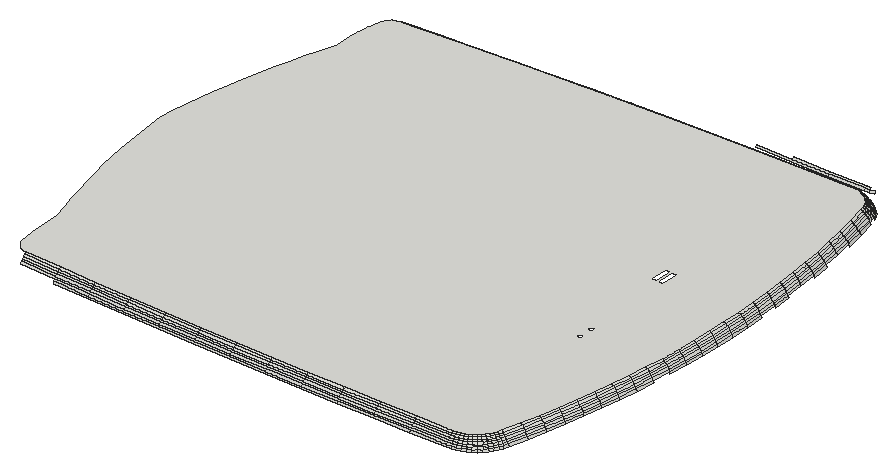
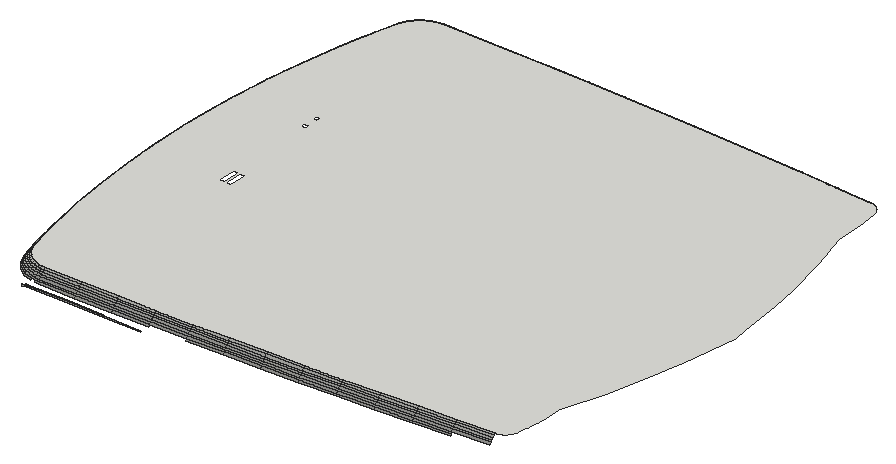
# SketchUp Ruby script. Lengths in inches.
U = 1.inch
M = Sketchup.active_model
def pt(a) = Geom::Point3d.new(a.map { |v| v * U })
def face(e, loops, mat)
  f = e.add_face(loops[0].map { |a| pt(a) })
  loops[1..].each { |l| e.add_face(l.map { |a| pt(a) }).erase! }
  f.material = f.back_material = mat if mat
  f
end
# faces: each face lists its corners as indices into pts; further lists are holes
def faces(e, pts, list, mat = nil) = list.each { |f| face(e, (f[0].is_a?(Array) ? f : [f]).map { |l| l.map { |i| pts[i] } }, mat) }
# xy, xz, yz: faces in a plane at the given z, y or x. An outline is a flat list of corners, or four numbers for a rectangle; further outlines are holes
def ring(l) = l.size == 4 ? [[l[0], l[1]], [l[2], l[1]], [l[2], l[3]], [l[0], l[3]]] : l.each_slice(2).to_a
def flat(e, list, mat, &to3) = list.each { |f| face(e, (f[0].is_a?(Array) ? f : [f]).map { |l| ring(l).map { |u, v| to3.(u, v) } }, mat) }
def xy(e, z, list, mat = nil) = flat(e, list, mat) { |x, y| [x, y, z] }
def xz(e, y, list, mat = nil) = flat(e, list, mat) { |x, z| [x, y, z] }
def yz(e, x, list, mat = nil) = flat(e, list, mat) { |y, z| [x, y, z] }
def lines(e, pts, list) = list.each { |a, b| e.add_line(pt(pts[a]), pt(pts[b])) }
# prism: a flat outline (further loops are holes) pulled along v
def prism(e, loops, v, mat = nil)
  f = face(e, loops, mat); d = Geom::Vector3d.new(v.map { |x| x * U })
  f.pushpull(f.normal.samedirection?(d) ? d.length : -d.length)
end
def box(e, o, s, mat = nil) = prism(e, [[o, [o[0] + s[0], o[1], o[2]], [o[0] + s[0], o[1] + s[1], o[2]], [o[0], o[1] + s[1], o[2]]]], [0, 0, s[2]], mat)
def at(x, y, z, deg = 0) = Geom::Transformation.translation(pt([x, y, z])) * Geom::Transformation.rotation(ORIGIN, Z_AXIS, deg.degrees)
def axes(o, x, y, z) = Geom::Transformation.new([*x, 0, *y, 0, *z, 0, *pt(o).to_a, 1])
def part(name) = M.definitions.add(name)
# library, detail: a bought-in or finely detailed component or shape, given as its bounding box
def library(name, o, s) = part(name).tap { |d| box(d.entities, o, s) }
def detail(e, o, s) = box(e.add_group.entities, o, s)
def put(e, d, t, mat = nil) = e.add_instance(d, t).tap { |i| i.material = mat if mat }
def group(e, t, mat = nil) = e.add_group.tap { |g| g.transformation = t; g.material = mat if mat }.entities
root = M.entities
xy(root,38.7,[[[351.193,51.843,351.37,51.853,351.53,51.881,351.686,51.926,351.836,51.99,351.977,52.07,352.109,52.166,352.228,52.276,352.335,52.399,352.426,52.533,352.502,52.677,352.56,52.829,352.608,53.01,352.823,53.897,353.02,54.788,353.199,55.682,353.359,56.58,353.5,57.481,353.623,58.385,353.726,59.291,353.811,60.199,353.878,61.109,353.925,62.019,353.953,62.931,353.963,63.843,353.953,64.755,353.925,65.666,353.878,66.577,353.811,67.487,353.726,68.395,353.623,69.301,353.5,70.205,353.359,71.106,353.199,72.004,353.02,72.898,352.823,73.788,352.608,74.676,352.56,74.857,352.502,75.009,352.426,75.152,352.335,75.287,352.228,75.41,352.109,75.52,351.977,75.616,351.836,75.696,351.686,75.759,351.53,75.805,351.37,75.833,351.193,75.843,349.441,75.838,347.676,75.824,345.91,75.801,344.144,75.768,342.379,75.726,340.614,75.675,340.613,75.675,338.849,75.615,337.085,75.545,335.321,75.465,333.557,75.377,331.794,75.279,330.048,75.173,329.964,75.162,329.891,75.144,329.82,75.119,329.753,75.086,329.689,75.046,329.63,75,329.576,74.948,329.527,74.891,329.486,74.828,329.451,74.762,329.423,74.692,329.4,74.61,329.364,74.437,329.33,74.254,329.3,74.07,329.275,73.885,329.255,73.7,329.239,73.514,329.228,73.328,329.221,73.141,329.218,72.955,329.221,72.768,329.227,72.582,329.245,72.297,328.999,71.521,328.795,70.834,328.605,70.144,328.428,69.449,328.265,68.752,328.115,68.051,327.978,67.348,327.855,66.642,327.745,65.934,327.649,65.224,327.567,64.513,327.502,63.843,327.567,63.173,327.649,62.461,327.745,61.751,327.855,61.043,327.978,60.338,328.115,59.634,328.265,58.934,328.428,58.236,328.605,57.542,328.795,56.851,328.999,56.165,329.245,55.389,329.227,55.104,329.221,54.917,329.218,54.731,329.221,54.544,329.228,54.358,329.239,54.172,329.255,53.986,329.275,53.801,329.3,53.616,329.33,53.432,329.364,53.249,329.4,53.076,329.423,52.994,329.451,52.924,329.486,52.858,329.527,52.795,329.576,52.738,329.63,52.685,329.689,52.639,329.753,52.6,329.82,52.567,329.891,52.542,329.964,52.524,330.048,52.513,331.794,52.407,333.557,52.309,335.321,52.22,337.085,52.141,338.849,52.071,340.614,52.011,342.379,51.959,344.144,51.917,345.91,51.885,347.676,51.861,349.441,51.847],[350.05,65.612,350.3,66.487],[349.737,65.612,349.987,66.487],[350.378,61.08,350.346,61.085,350.316,61.097,350.29,61.117,350.27,61.143,350.258,61.173,350.253,61.205,350.258,61.238,350.27,61.268,350.29,61.294,350.316,61.314,350.346,61.326,350.378,61.33,350.411,61.326,350.441,61.314,350.467,61.294,350.487,61.268,350.499,61.238,350.503,61.205,350.499,61.173,350.487,61.143,350.467,61.117,350.441,61.097,350.411,61.085],[350.377,60.377,350.344,60.382,350.314,60.394,350.288,60.414,350.268,60.44,350.256,60.47,350.252,60.502,350.256,60.535,350.268,60.565,350.288,60.591,350.314,60.611,350.344,60.623,350.377,60.627,350.409,60.623,350.439,60.611,350.465,60.591,350.485,60.565,350.497,60.535,350.502,60.502,350.497,60.47,350.485,60.44,350.465,60.414,350.439,60.394,350.409,60.382]]])
p = [[349.439,51.479,38.259],[349.439,51.44,38.171],[347.671,51.454,38.171],[347.672,51.493,38.259],[351.204,51.475,38.259],[351.205,51.435,38.171],
  [351.412,51.487,38.259],[351.416,51.447,38.171],[351.613,51.522,38.259],[351.622,51.483,38.171],[344.137,51.549,38.259],[344.136,51.51,38.171],
  [342.368,51.552,38.171],[342.369,51.592,38.259],[345.904,51.517,38.259],[345.903,51.477,38.171],[351.81,51.579,38.259],[351.823,51.542,38.171],
  [351.998,51.659,38.259],[352.016,51.624,38.171],[340.602,51.643,38.259],[340.601,51.603,38.171],[338.834,51.664,38.171],[338.836,51.704,38.259],
  [352.177,51.76,38.259],[352.198,51.727,38.171],[337.069,51.774,38.259],[337.068,51.734,38.171],[335.301,51.813,38.171],[335.303,51.853,38.259],
  [352.342,51.881,38.259],[352.367,51.85,38.171],[333.536,51.902,38.171],[333.538,51.942,38.259],[352.493,52.019,38.259],[352.521,51.992,38.171],
  [331.77,52,38.171],[331.773,52.04,38.259],[352.627,52.174,38.259],[352.658,52.15,38.171],[352.742,52.344,38.259],[352.776,52.323,38.171],
  [352.837,52.525,38.259],[352.874,52.508,38.171],[352.911,52.716,38.259],[352.949,52.704,38.171],[352.964,52.92,38.259],[353.003,52.91,38.171],
  [353.182,53.814,38.259],[353.221,53.805,38.171],[353.38,54.712,38.259],[353.419,54.704,38.171],[353.56,55.614,38.259],[353.6,55.607,38.171],
  [353.722,56.519,38.259],[353.761,56.513,38.171],[353.864,57.428,38.259],[353.904,57.422,38.171],[353.988,58.339,38.259],[354.027,58.334,38.171],
  [354.092,59.253,38.259],[354.132,59.249,38.171],[354.178,60.168,38.259],[354.218,60.165,38.171],[354.292,62.004,38.259],[354.332,62.002,38.171],
  [354.285,61.083,38.171],[354.245,61.086,38.259],[354.321,62.923,38.259],[354.361,62.922,38.171],[354.331,63.843,38.259],[354.37,63.843,38.171],
  [354.321,64.762,38.259],[354.361,64.763,38.171],[354.292,65.682,38.259],[354.332,65.683,38.171],[354.245,66.6,38.259],[354.285,66.603,38.171],
  [354.092,68.433,38.259],[354.132,68.437,38.171],[354.218,67.521,38.171],[354.178,67.517,38.259],[353.722,71.166,38.259],[353.761,71.173,38.171],
  [353.904,70.264,38.171],[353.864,70.258,38.259],[353.182,73.872,38.259],[353.221,73.881,38.171],[353.419,72.982,38.171],[353.38,72.974,38.259],
  [352.964,74.766,38.259],[353.003,74.775,38.171],[352.742,75.342,38.259],[352.776,75.363,38.171],[352.874,75.177,38.171],[352.837,75.161,38.259],
  [352.627,75.511,38.259],[352.658,75.536,38.171],[352.493,75.666,38.259],[352.521,75.694,38.171],[331.773,75.646,38.259],[331.77,75.686,38.171],
  [333.536,75.784,38.171],[333.538,75.744,38.259],[335.301,75.873,38.171],[335.303,75.833,38.259],[352.342,75.805,38.259],[352.367,75.836,38.171],
  [337.068,75.952,38.171],[337.069,75.912,38.259],[352.177,75.926,38.259],[352.198,75.959,38.171],[338.834,76.022,38.171],[338.836,75.982,38.259],
  [351.998,76.026,38.259],[352.016,76.062,38.171],[340.601,76.083,38.171],[340.602,76.043,38.259],[342.368,76.134,38.171],[342.369,76.094,38.259],
  [351.81,76.106,38.259],[351.823,76.144,38.171],[344.136,76.176,38.171],[344.137,76.136,38.259],[351.613,76.164,38.259],[351.622,76.203,38.171],
  [345.904,76.169,38.259],[345.903,76.209,38.171],[347.671,76.232,38.171],[347.672,76.192,38.259],[349.439,76.246,38.171],[349.439,76.206,38.259],
  [351.205,76.251,38.171],[351.204,76.211,38.259],[351.416,76.239,38.171],[351.412,76.199,38.259],[347.672,76.743,38.259],[347.671,76.704,38.171],
  [345.903,76.727,38.171],[345.904,76.767,38.259],[349.439,76.729,38.259],[349.439,76.69,38.171],[351.204,76.725,38.259],[351.205,76.685,38.171],
  [351.412,76.737,38.259],[351.416,76.697,38.171],[351.613,76.772,38.259],[351.622,76.733,38.171],[344.138,51.596,38.344],[342.371,51.638,38.344],
  [345.905,51.563,38.344],[347.672,51.54,38.344],[347.673,51.593,38.424],[345.906,51.616,38.424],[349.44,51.526,38.344],[349.44,51.579,38.424],
  [351.202,51.521,38.344],[351.201,51.574,38.424],[351.406,51.533,38.344],[351.4,51.586,38.424],[351.603,51.567,38.344],[351.591,51.619,38.424],
  [351.794,51.623,38.344],[340.604,51.689,38.344],[338.837,51.75,38.344],[342.372,51.691,38.424],[340.605,51.742,38.424],[344.139,51.649,38.424],
  [351.776,51.673,38.424],[351.978,51.701,38.344],[351.954,51.749,38.424],[337.071,51.82,38.344],[338.839,51.803,38.424],[337.073,51.873,38.424],
  [352.151,51.799,38.344],[352.123,51.844,38.424],[335.305,51.899,38.344],[335.308,51.952,38.424],[352.279,51.958,38.424],[352.3125,51.917,38.344],
  [333.54,51.988,38.344],[331.775,52.086,38.344],[333.543,52.041,38.424],[352.459,52.052,38.344],[352.421,52.089,38.424],[331.778,52.139,38.424],
  [352.59,52.203,38.344],[330.017,52.193,38.344],[330.022,52.246,38.424],[352.548,52.235,38.424],[352.657,52.395,38.424],[352.702,52.367,38.344],
  [352.795,52.544,38.344],[352.747,52.566,38.424],[352.816,52.746,38.424],[352.867,52.73,38.344],[352.868,52.944,38.424],[352.919,52.932,38.344],
  [353.136,53.825,38.344],[353.085,53.837,38.424],[353.335,54.722,38.344],[353.283,54.732,38.424],[353.515,55.623,38.344],[353.463,55.632,38.424],
  [353.676,56.527,38.344],[353.624,56.536,38.424],[353.766,57.442,38.424],[353.818,57.435,38.344],[353.942,58.345,38.344],[353.889,58.351,38.424],
  [354.046,59.258,38.344],[353.994,59.263,38.424],[354.132,60.172,38.344],[354.079,60.177,38.424],[354.198,61.089,38.344],[354.146,61.092,38.424],
  [354.193,62.008,38.424],[354.246,62.006,38.344],[354.275,62.924,38.344],[354.222,62.925,38.424],[354.231,63.843,38.424],[354.284,63.843,38.344],
  [354.222,64.76,38.424],[354.275,64.762,38.344],[354.193,65.678,38.424],[354.246,65.68,38.344],[354.146,66.594,38.424],[354.198,66.597,38.344],
  [354.079,67.509,38.424],[354.132,67.513,38.344],[353.994,68.423,38.424],[354.046,68.428,38.344],[353.889,69.334,38.424],[353.942,69.341,38.344],
  [353.988,69.347,38.259],[353.766,70.244,38.424],[353.818,70.251,38.344],[353.624,71.15,38.424],[353.676,71.159,38.344],[353.463,72.053,38.424],
  [353.515,72.063,38.344],[353.56,72.072,38.259],[353.283,72.953,38.424],[353.335,72.964,38.344],[353.085,73.849,38.424],[353.136,73.861,38.344],
  [352.868,74.741,38.424],[352.919,74.754,38.344],[352.816,74.939,38.424],[352.867,74.956,38.344],[352.911,74.97,38.259],[352.747,75.12,38.424],
  [352.795,75.142,38.344],[352.657,75.291,38.424],[352.702,75.318,38.344],[352.548,75.451,38.424],[352.59,75.483,38.344],[330.022,75.44,38.424],
  [330.017,75.493,38.344],[331.775,75.6,38.344],[331.778,75.547,38.424],[333.54,75.698,38.344],[333.543,75.645,38.424],[352.421,75.597,38.424],
  [352.459,75.634,38.344],[335.305,75.786,38.344],[335.308,75.734,38.424],[352.279,75.728,38.424],[352.3125,75.769,38.344],[337.071,75.866,38.344],
  [337.073,75.813,38.424],[352.123,75.842,38.424],[352.151,75.886,38.344],[338.837,75.936,38.344],[338.839,75.883,38.424],[351.954,75.937,38.424],
  [351.978,75.985,38.344],[340.603,75.996,38.344],[340.605,75.944,38.424],[342.371,76.048,38.344],[342.372,75.995,38.424],[351.776,76.013,38.424],
  [351.794,76.0625,38.344],[344.138,76.09,38.344],[344.139,76.037,38.424],[345.905,76.122,38.344],[345.906,76.07,38.424],[351.591,76.067,38.424],
  [351.603,76.119,38.344],[347.672,76.146,38.344],[347.673,76.093,38.424],[349.44,76.16,38.344],[349.44,76.107,38.424],[351.202,76.164,38.344],
  [351.201,76.112,38.424],[351.406,76.153,38.344],[351.4,76.1,38.424],[349.44,76.776,38.344],[347.672,76.79,38.344],[351.202,76.771,38.344],
  [351.406,76.783,38.344],[344.14,51.708,38.501],[342.374,51.75,38.501],[345.907,51.675,38.501],[347.673,51.652,38.501],[349.44,51.638,38.501],
  [351.199,51.633,38.501],[351.393,51.644,38.501],[351.577,51.676,38.501],[351.756,51.729,38.501],[340.607,51.801,38.501],[338.841,51.862,38.501],
  [351.928,51.802,38.501],[352.091,51.893,38.501],[337.076,51.932,38.501],[352.242,52.003,38.501],[335.311,52.011,38.501],[333.546,52.1,38.501],
  [331.782,52.198,38.501],[352.379,52.13,38.501],[330.028,52.304,38.501],[352.501,52.271,38.501],[352.606,52.425,38.501],[352.693,52.59,38.501],
  [352.76,52.764,38.501],[352.811,52.959,38.501],[353.028,53.85,38.501],[353.226,54.745,38.501],[353.405,55.643,38.501],[353.566,56.545,38.501],
  [353.708,57.451,38.501],[353.831,58.359,38.501],[353.935,59.269,38.501],[354.02,60.182,38.501],[354.087,61.096,38.501],[354.134,62.011,38.501],
  [354.163,62.927,38.501],[354.172,63.843,38.501],[354.163,64.759,38.501],[354.134,65.675,38.501],[354.087,66.59,38.501],[354.02,67.504,38.501],
  [353.935,68.417,38.501],[353.831,69.327,38.501],[353.708,70.235,38.501],[353.566,71.14,38.501],[353.405,72.042,38.501],[353.226,72.941,38.501],
  [353.028,73.836,38.501],[352.811,74.727,38.501],[352.76,74.921,38.501],[352.693,75.095,38.501],[352.606,75.261,38.501],[352.501,75.415,38.501],
  [330.028,75.381,38.501],[331.782,75.488,38.501],[352.379,75.556,38.501],[333.546,75.586,38.501],[335.311,75.675,38.501],[352.242,75.682,38.501],
  [337.076,75.754,38.501],[352.091,75.792,38.501],[338.841,75.824,38.501],[340.607,75.885,38.501],[351.928,75.884,38.501],[342.374,75.936,38.501],
  [344.14,75.978,38.501],[351.756,75.957,38.501],[345.907,76.011,38.501],[347.673,76.034,38.501],[349.44,76.048,38.501],[351.199,76.053,38.501],
  [351.393,76.042,38.501],[351.577,76.01,38.501],[349.441,51.702,38.573],[347.674,51.716,38.573],[351.197,51.698,38.573],[351.386,51.709,38.573],
  [351.5625,51.739,38.573],[342.375,51.814,38.573],[340.609,51.866,38.573],[344.141,51.772,38.573],[345.908,51.74,38.573],[351.735,51.79,38.573],
  [351.9,51.86,38.573],[338.844,51.926,38.573],[352.056,51.948,38.573],[337.079,51.996,38.573],[335.314,52.076,38.573],[352.201,52.053,38.573],
  [333.549,52.164,38.573],[352.332,52.175,38.573],[331.786,52.262,38.573],[352.45,52.31,38.573],[330.034,52.369,38.573],[352.551,52.459,38.573],
  [352.634,52.617,38.573],[352.699,52.784,38.573],[352.748,52.975,38.573],[352.965,53.865,38.573],[353.162,54.758,38.573],[353.341,55.655,38.573],
  [353.502,56.556,38.573],[353.644,57.46,38.573],[353.767,58.367,38.573],[353.871,59.276,38.573],[353.956,60.187,38.573],[354.022,61.1,38.573],
  [354.07,62.013,38.573],[354.098,62.928,38.573],[354.108,63.843,38.573],[354.098,64.758,38.573],[354.07,65.672,38.573],[354.022,66.586,38.573],
  [353.956,67.499,38.573],[353.871,68.41,38.573],[353.767,69.319,38.573],[353.644,70.226,38.573],[353.502,71.13,38.573],[353.341,72.03,38.573],
  [353.162,72.928,38.573],[352.965,73.821,38.573],[352.748,74.711,38.573],[352.699,74.901,38.573],[352.634,75.069,38.573],[352.551,75.227,38.573],
  [352.45,75.375,38.573],[330.034,75.317,38.573],[331.786,75.424,38.573],[333.549,75.522,38.573],[352.332,75.511,38.573],[335.314,75.61,38.573],
  [352.201,75.632,38.573],[337.079,75.689,38.573],[352.056,75.738,38.573],[338.844,75.759,38.573],[351.9,75.826,38.573],[340.608,75.82,38.573],
  [342.375,75.871,38.573],[351.735,75.896,38.573],[344.141,75.913,38.573],[345.908,75.946,38.573],[347.674,75.969,38.573],[351.386,75.977,38.573],
  [351.5625,75.947,38.573],[349.441,75.983,38.573],[351.197,75.988,38.573],[345.909,51.81,38.639],[344.143,51.842,38.639],[347.675,51.786,38.639],
  [349.441,51.772,38.639],[351.196,51.768,38.639],[351.378,51.778,38.639],[351.547,51.807,38.639],[351.711,51.856,38.639],[342.377,51.884,38.639],
  [340.612,51.936,38.639],[344.144,51.917,38.7],[342.379,51.959,38.7],[345.91,51.885,38.7],[347.676,51.861,38.7],[349.441,51.847,38.7],
  [351.193,51.843,38.7],[351.37,51.853,38.7],[351.53,51.881,38.7],[351.686,51.926,38.7],[351.869,51.923,38.639],[338.846,51.996,38.639],
  [337.082,52.066,38.639],[340.614,52.011,38.7],[338.849,52.071,38.7],[351.836,51.99,38.7],[351.977,52.07,38.7],[352.018,52.007,38.639],
  [352.156,52.108,38.639],[335.317,52.146,38.639],[337.085,52.141,38.7],[352.109,52.166,38.7],[333.553,52.234,38.639],[335.321,52.22,38.7],
  [333.557,52.309,38.7],[352.228,52.276,38.7],[352.282,52.224,38.639],[331.79,52.332,38.639],[331.794,52.407,38.7],[352.335,52.399,38.7],
  [352.394,52.353,38.639],[330.041,52.438,38.639],[330.048,52.513,38.7],[352.49,52.495,38.639],[352.426,52.533,38.7],[352.502,52.677,38.7],
  [352.57,52.646,38.639],[352.56,52.829,38.7],[352.632,52.806,38.639],[352.68,52.992,38.639],[352.608,53.01,38.7],[352.823,53.897,38.7],
  [352.896,53.88,38.639],[353.02,54.788,38.7],[353.094,54.772,38.639],[353.199,55.682,38.7],[353.273,55.668,38.639],[353.359,56.58,38.7],
  [353.433,56.568,38.639],[353.574,57.47,38.639],[353.5,57.481,38.7],[353.623,58.385,38.7],[353.697,58.375,38.639],[353.726,59.291,38.7],
  [353.801,59.283,38.639],[353.811,60.199,38.7],[353.886,60.193,38.639],[353.878,61.109,38.7],[353.952,61.104,38.639],[353.925,62.019,38.7],
  [354,62.016,38.639],[353.953,62.931,38.7],[354.028,62.929,38.639],[354.038,63.843,38.639],[353.963,63.843,38.7],[353.953,64.755,38.7],
  [354.028,64.756,38.639],[353.925,65.666,38.7],[354,65.67,38.639],[353.878,66.577,38.7],[353.952,66.582,38.639],[353.811,67.487,38.7],
  [353.886,67.493,38.639],[353.726,68.395,38.7],[353.801,68.403,38.639],[353.623,69.301,38.7],[353.697,69.31,38.639],[353.5,70.205,38.7],
  [353.574,70.216,38.639],[353.359,71.106,38.7],[353.433,71.118,38.639],[353.199,72.004,38.7],[353.273,72.017,38.639],[353.02,72.898,38.7],
  [353.094,72.913,38.639],[352.823,73.788,38.7],[352.896,73.805,38.639],[352.608,74.676,38.7],[352.68,74.694,38.639],[352.56,74.857,38.7],
  [352.632,74.88,38.639],[352.502,75.009,38.7],[352.57,75.04,38.639],[352.426,75.152,38.7],[352.49,75.191,38.639],[330.048,75.173,38.7],
  [330.041,75.247,38.639],[331.79,75.354,38.639],[331.794,75.279,38.7],[352.335,75.287,38.7],[352.394,75.333,38.639],[333.553,75.452,38.639],
  [333.557,75.377,38.7],[352.228,75.41,38.7],[352.282,75.462,38.639],[335.317,75.54,38.639],[335.321,75.465,38.7],[352.109,75.52,38.7],
  [352.156,75.578,38.639],[337.082,75.619,38.639],[337.085,75.545,38.7],[338.846,75.689,38.639],[338.849,75.615,38.7],[351.977,75.616,38.7],
  [352.018,75.679,38.639],[340.61,75.75,38.639],[340.613,75.675,38.7],[351.836,75.696,38.7],[351.869,75.763,38.639],[342.379,75.726,38.7],
  [340.614,75.675,38.7],[340.612,75.75,38.639],[342.377,75.801,38.639],[344.143,75.843,38.639],[344.144,75.768,38.7],[351.686,75.759,38.7],
  [351.711,75.83,38.639],[345.909,75.876,38.639],[345.91,75.801,38.7],[347.675,75.899,38.639],[347.676,75.824,38.7],[349.441,75.913,38.639],
  [349.441,75.838,38.7],[351.196,75.918,38.639],[351.193,75.843,38.7],[351.378,75.908,38.639],[351.37,75.833,38.7],[351.547,75.878,38.639],
  [351.53,75.805,38.7]]
faces(root,p,[[0,1,2,3],[4,5,1,0],[6,7,5,4],[8,9,7,6],[10,11,12,13],[14,15,11,10],[3,2,15,14],[16,17,9,8],
  [18,19,17,16],[20,21,22,23],[13,12,21,20],[24,25,19,18],[26,27,28,29],[23,22,27,26],[30,31,25,24],[29,28,32,33],
  [34,35,31,30],[33,32,36,37],[38,39,35,34],[40,41,39,38],[42,43,41,40],[44,45,43,42],[46,47,45,44],[48,49,47,46],
  [50,51,49,48],[52,53,51,50],[54,55,53,52],[56,57,55,54],[58,59,57,56],[60,61,59,58],[62,63,61,60],[64,65,66,67],
  [68,69,65,64],[70,71,69,68],[72,73,71,70],[74,75,73,72],[76,77,75,74],[78,79,80,81],[82,83,84,85],[86,87,88,89],
  [90,91,87,86],[92,93,94,95],[96,97,93,92],[98,99,97,96],[100,101,102,103],[103,102,104,105],[106,107,99,98],[105,104,108,109],
  [110,111,107,106],[109,108,112,113],[114,115,111,110],[113,112,116,117],[117,116,118,119],[120,121,115,114],[119,118,122,123],[124,125,121,120],
  [126,127,128,129],[129,128,130,131],[131,130,132,133],[133,132,134,135],[136,137,138,139],[140,141,137,136],[142,143,141,140],[144,145,143,142],
  [146,147,145,144],[148,10,13,149],[150,14,10,148],[151,3,14,150],[152,151,150,153],[154,0,3,151],[155,154,151,152],[156,4,0,154],
  [157,156,154,155],[158,6,4,156],[159,158,156,157],[160,8,6,158],[161,160,158,159],[162,16,8,160],[163,20,23,164],[149,13,20,163],
  [165,149,163,166],[167,148,149,165],[153,150,148,167],[168,162,160,161],[169,18,16,162],[170,169,162,168],[164,23,26,171],[172,164,171,173],
  [166,163,164,172],[174,24,18,169],[175,174,169,170],[171,26,29,176],[173,171,176,177],[178,179,174,175],[179,30,24,174],[180,33,37,181],
  [176,29,33,180],[177,176,180,182],[183,34,30,179],[184,183,179,178],[182,180,181,185],[186,38,34,183],[185,181,187,188],[189,186,183,184],
  [190,191,186,189],[191,40,38,186],[192,42,40,191],[193,192,191,190],[194,195,192,193],[195,44,42,192],[196,197,195,194],[197,46,44,195],
  [198,48,46,197],[199,198,197,196],[200,50,48,198],[201,200,198,199],[202,52,50,200],[203,202,200,201],[204,54,52,202],[205,204,202,203],
  [206,207,204,205],[207,56,54,204],[208,58,56,207],[209,208,207,206],[210,60,58,208],[211,210,208,209],[212,62,60,210],[213,212,210,211],
  [214,67,62,212],[215,214,212,213],[216,217,214,215],[217,64,67,214],[218,68,64,217],[219,218,217,216],[220,221,218,219],[221,70,68,218],
  [222,223,221,220],[223,72,70,221],[224,225,223,222],[225,74,72,223],[226,227,225,224],[227,76,74,225],[228,229,227,226],[229,81,76,227],
  [230,231,229,228],[231,78,81,229],[232,233,231,230],[233,234,78,231],[235,236,233,232],[236,85,234,233],[237,238,236,235],[238,82,85,236],
  [239,240,238,237],[240,241,82,238],[242,243,240,239],[243,89,241,240],[244,245,243,242],[245,86,89,243],[246,247,245,244],[247,90,86,245],
  [248,249,247,246],[249,250,90,247],[251,252,249,248],[252,95,250,249],[253,254,252,251],[254,92,95,252],[255,256,254,253],[256,96,92,254],
  [257,258,259,260],[260,259,261,262],[263,264,256,255],[264,98,96,256],[259,100,103,261],[262,261,265,266],[267,268,264,263],[268,106,98,264],
  [261,103,105,265],[266,265,269,270],[271,272,268,267],[265,105,109,269],[270,269,273,274],[275,276,272,271],[272,110,106,268],[269,109,113,273],
  [274,273,277,278],[273,113,117,277],[278,277,279,280],[281,282,276,275],[276,114,110,272],[277,117,119,279],[280,279,283,284],[279,119,123,283],
  [284,283,285,286],[287,288,282,281],[282,120,114,276],[283,123,126,285],[286,285,289,290],[285,126,129,289],[290,289,291,292],[289,129,131,291],
  [292,291,293,294],[294,293,295,296],[296,295,288,287],[295,135,124,288],[288,124,120,282],[291,131,133,293],[293,133,135,295],[297,140,136,298],
  [299,142,140,297],[300,144,142,299],[301,167,165,302],[303,153,167,301],[304,152,153,303],[305,155,152,304],[306,157,155,305],[307,159,157,306],
  [308,161,159,307],[309,168,161,308],[310,166,172,311],[302,165,166,310],[312,170,168,309],[313,175,170,312],[311,172,173,314],[315,178,175,313],
  [314,173,177,316],[317,182,185,318],[316,177,182,317],[319,184,178,315],[318,185,188,320],[321,189,184,319],[322,190,189,321],[323,193,190,322],
  [324,194,193,323],[325,196,194,324],[326,199,196,325],[327,201,199,326],[328,203,201,327],[329,205,203,328],[330,206,205,329],[331,209,206,330],
  [332,211,209,331],[333,213,211,332],[334,215,213,333],[335,216,215,334],[336,219,216,335],[337,220,219,336],[338,222,220,337],[339,224,222,338],
  [340,226,224,339],[341,228,226,340],[342,230,228,341],[343,232,230,342],[344,235,232,343],[345,237,235,344],[346,239,237,345],[347,242,239,346],
  [348,244,242,347],[349,246,244,348],[350,248,246,349],[351,251,248,350],[352,253,251,351],[353,255,253,352],[354,257,260,355],[356,263,255,353],
  [355,260,262,357],[357,262,266,358],[359,267,263,356],[358,266,270,360],[361,271,267,359],[360,270,274,362],[362,274,278,363],[364,275,271,361],
  [363,278,280,365],[365,280,284,366],[367,281,275,364],[366,284,286,368],[368,286,290,369],[369,290,292,370],[370,292,294,371],[371,294,296,372],
  [372,296,287,373],[373,287,281,367],[374,305,304,375],[376,306,305,374],[377,307,306,376],[378,308,307,377],[379,302,310,380],[381,301,302,379],
  [382,303,301,381],[375,304,303,382],[383,309,308,378],[384,312,309,383],[380,310,311,385],[386,313,312,384],[387,314,316,388],[385,311,314,387],
  [389,315,313,386],[388,316,317,390],[391,319,315,389],[390,317,318,392],[393,321,319,391],[392,318,320,394],[395,322,321,393],[396,323,322,395],
  [397,324,323,396],[398,325,324,397],[399,326,325,398],[400,327,326,399],[401,328,327,400],[402,329,328,401],[403,330,329,402],[404,331,330,403],
  [405,332,331,404],[406,333,332,405],[407,334,333,406],[408,335,334,407],[409,336,335,408],[410,337,336,409],[411,338,337,410],[412,339,338,411],
  [413,340,339,412],[414,341,340,413],[415,342,341,414],[416,343,342,415],[417,344,343,416],[418,345,344,417],[419,346,345,418],[420,347,346,419],
  [421,348,347,420],[422,349,348,421],[423,350,349,422],[424,351,350,423],[425,352,351,424],[426,353,352,425],[427,354,355,428],[428,355,357,429],
  [430,356,353,426],[429,357,358,431],[432,359,356,430],[431,358,360,433],[434,361,359,432],[433,360,362,435],[436,364,361,434],[435,362,363,437],
  [437,363,365,438],[439,367,364,436],[438,365,366,440],[440,366,368,441],[441,368,369,442],[443,372,373,444],[444,373,367,439],[442,369,370,445],
  [445,370,371,446],[446,371,372,443],[447,382,381,448],[449,375,382,447],[450,374,375,449],[451,376,374,450],[452,377,376,451],[453,378,377,452],
  [454,383,378,453],[455,379,380,456],[448,381,379,455],[457,448,455,458],[459,447,448,457],[460,449,447,459],[461,450,449,460],[462,451,450,461],
  [463,452,451,462],[464,453,452,463],[465,454,453,464],[466,384,383,454],[467,385,387,468],[456,380,385,467],[469,456,467,470],[458,455,456,469],
  [471,466,454,465],[472,473,466,471],[473,386,384,466],[474,389,386,473],[468,387,388,475],[470,467,468,476],[477,474,473,472],[475,388,390,478],
  [479,475,478,480],[476,468,475,479],[481,482,474,477],[482,391,389,474],[478,390,392,483],[480,478,483,484],[485,486,482,481],[486,393,391,482],
  [483,392,394,487],[484,483,487,488],[489,395,393,486],[490,489,486,485],[491,492,489,490],[492,396,395,489],[493,494,492,491],[494,397,396,492],
  [495,398,397,494],[496,495,494,493],[497,498,495,496],[498,399,398,495],[499,500,498,497],[500,400,399,498],[501,502,500,499],[502,401,400,500],
  [503,504,502,501],[504,402,401,502],[505,403,402,504],[506,505,504,503],[507,508,505,506],[508,404,403,505],[509,510,508,507],[510,405,404,508],
  [511,512,510,509],[512,406,405,510],[513,514,512,511],[514,407,406,512],[515,516,514,513],[516,408,407,514],[517,518,516,515],[518,409,408,516],
  [519,410,409,518],[520,519,518,517],[521,522,519,520],[522,411,410,519],[523,524,522,521],[524,412,411,522],[525,526,524,523],[526,413,412,524],
  [527,528,526,525],[528,414,413,526],[529,530,528,527],[530,415,414,528],[531,532,530,529],[532,416,415,530],[533,534,532,531],[534,417,416,532],
  [535,536,534,533],[536,418,417,534],[537,538,536,535],[538,419,418,536],[539,540,538,537],[540,420,419,538],[541,542,540,539],[542,421,420,540],
  [543,544,542,541],[544,422,421,542],[545,546,544,543],[546,423,422,544],[547,548,546,545],[548,424,423,546],[549,550,548,547],[550,425,424,548],
  [551,552,553,554],[552,427,428,553],[555,556,550,549],[556,426,425,550],[554,553,557,558],[559,560,556,555],[560,430,426,556],[553,428,429,557],
  [558,557,561,562],[563,564,560,559],[557,429,431,561],[562,561,565,566],[561,431,433,565],[566,565,567,568],[569,570,564,563],[564,432,430,560],
  [565,433,435,567],[567,571,572,568],[573,574,570,569],[570,434,432,564],[435,437,571,567],[575,576,577,578],[575,578,579,580],[581,582,574,573],
  [574,436,434,570],[578,577,437,438],[578,438,440,579],[580,579,583,584],[579,440,441,583],[584,583,585,586],[586,585,587,588],[588,587,589,590],
  [590,589,591,592],[592,591,593,594],[594,593,582,581],[593,444,439,582],[582,439,436,574],[583,441,442,585],[585,442,445,587],[587,445,446,589],
  [589,446,443,591],[591,443,444,593]])
